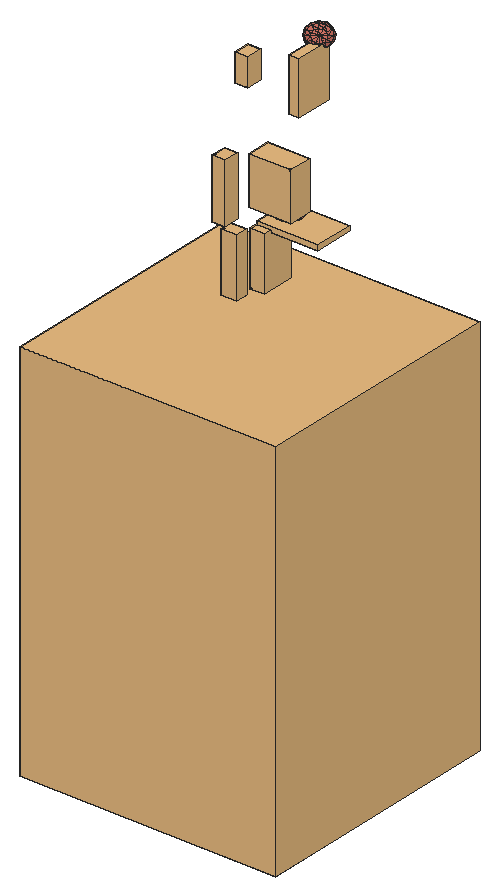
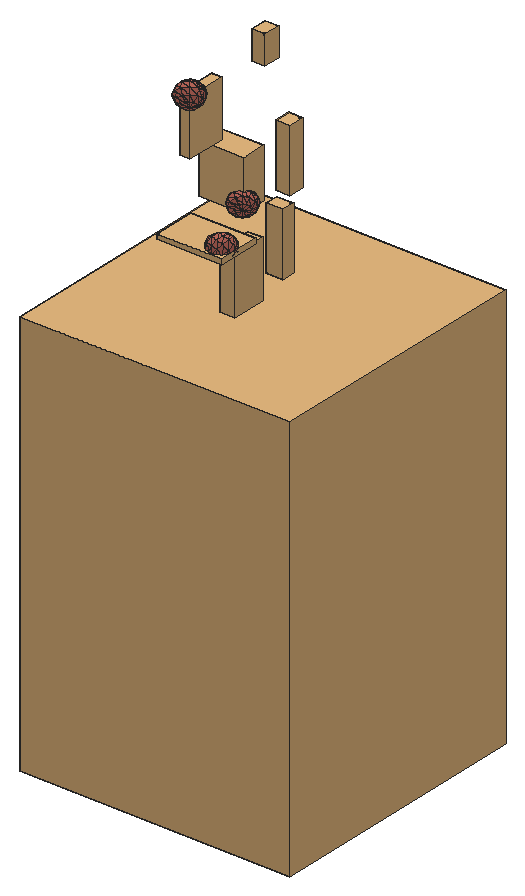
# SketchUp Ruby script. Lengths in inches.
U = 1.inch
M = Sketchup.active_model
def pt(a) = Geom::Point3d.new(a.map { |v| v * U })
def face(e, loops, mat)
  f = e.add_face(loops[0].map { |a| pt(a) })
  loops[1..].each { |l| e.add_face(l.map { |a| pt(a) }).erase! }
  f.material = f.back_material = mat if mat
  f
end
# faces: each face lists its corners as indices into pts; further lists are holes
def faces(e, pts, list, mat = nil) = list.each { |f| face(e, (f[0].is_a?(Array) ? f : [f]).map { |l| l.map { |i| pts[i] } }, mat) }
# xy, xz, yz: faces in a plane at the given z, y or x. An outline is a flat list of corners, or four numbers for a rectangle; further outlines are holes
def ring(l) = l.size == 4 ? [[l[0], l[1]], [l[2], l[1]], [l[2], l[3]], [l[0], l[3]]] : l.each_slice(2).to_a
def flat(e, list, mat, &to3) = list.each { |f| face(e, (f[0].is_a?(Array) ? f : [f]).map { |l| ring(l).map { |u, v| to3.(u, v) } }, mat) }
def xy(e, z, list, mat = nil) = flat(e, list, mat) { |x, y| [x, y, z] }
def xz(e, y, list, mat = nil) = flat(e, list, mat) { |x, z| [x, y, z] }
def yz(e, x, list, mat = nil) = flat(e, list, mat) { |y, z| [x, y, z] }
def lines(e, pts, list) = list.each { |a, b| e.add_line(pt(pts[a]), pt(pts[b])) }
# prism: a flat outline (further loops are holes) pulled along v
def prism(e, loops, v, mat = nil)
  f = face(e, loops, mat); d = Geom::Vector3d.new(v.map { |x| x * U })
  f.pushpull(f.normal.samedirection?(d) ? d.length : -d.length)
end
def box(e, o, s, mat = nil) = prism(e, [[o, [o[0] + s[0], o[1], o[2]], [o[0] + s[0], o[1] + s[1], o[2]], [o[0], o[1] + s[1], o[2]]]], [0, 0, s[2]], mat)
def at(x, y, z, deg = 0) = Geom::Transformation.translation(pt([x, y, z])) * Geom::Transformation.rotation(ORIGIN, Z_AXIS, deg.degrees)
def axes(o, x, y, z) = Geom::Transformation.new([*x, 0, *y, 0, *z, 0, *pt(o).to_a, 1])
def part(name) = M.definitions.add(name)
# library, detail: a bought-in or finely detailed component or shape, given as its bounding box
def library(name, o, s) = part(name).tap { |d| box(d.entities, o, s) }
def detail(e, o, s) = box(e.add_group.entities, o, s)
def put(e, d, t, mat = nil) = e.add_instance(d, t).tap { |i| i.material = mat if mat }
def group(e, t, mat = nil) = e.add_group.tap { |g| g.transformation = t; g.material = mat if mat }.entities
root = M.entities
M.materials.add("green").color = [174, 139, 102]
M.materials.add("st tile").color = [196, 179, 155]
M.materials.add("vio").color = [206, 114, 100]
c1 = library("3DGeom~165_Defintion",[-129.92,-500,-108.02],[259.84,1000,216.04])
c2 = part("3DGeom~166_Defintion")
p = [[102.48,500,-82.55],[119.68,491.3,-106.9],[111.55,493.01,-108.02],[102.48,500,-82.55],[111.55,493.01,-108.02],[104.2,495.34,-104.9],
  [102.48,500,-82.55],[126.4,490.68,-101.84],[119.68,491.3,-106.9],[102.48,500,-82.55],[104.2,495.34,-104.9],[99.59,497.67,-98.37],
  [102.48,500,-82.55],[129.92,491.3,-94.2],[126.4,490.68,-101.84],[102.48,500,-82.55],[99.59,497.67,-98.37],[98.96,499.375,-90.19],
  [102.48,500,-82.55],[129.29,493.01,-86.02],[129.92,491.3,-94.2],[102.48,500,-82.55],[124.6875,495.34,-79.5],[129.29,493.01,-86.02],
  [102.48,500,-82.55],[117.33,497.67,-76.375],[124.6875,495.34,-79.5],[102.48,500,-82.55],[109.21,499.375,-77.49],[117.33,497.67,-76.375],
  [-108.37,-495.57,69.37],[-118.11,-500,95.38],[-120.78,-498.52,79.375],[-93.3,-494.09,75.36],[-118.11,-500,95.38],[-108.37,-495.57,69.37],
  [-108.37,-495.57,69.37],[-120.78,-498.52,79.375],[-115.95,-497.04,72.67],[-93.3,-494.09,75.36],[-108.37,-495.57,69.37],[-100.08,-494.49,70.35],
  [-90.63,-495.57,91.37],[-118.11,-500,95.38],[-93.3,-494.09,75.36],[-90.63,-495.57,91.37],[-93.3,-494.09,75.36],[-89.84,-494.49,83.05],
  [-118.11,-500,95.38],[-121.57,-499.6,87.6875],[-120.78,-498.52,79.375],[-103.04,-498.52,101.375],[-118.11,-500,95.38],[-90.63,-495.57,91.37],
  [-103.04,-498.52,101.375],[-90.63,-495.57,91.37],[-95.46,-497.04,98.07],[-118.11,-500,95.38],[-103.04,-498.52,101.375],[-111.33,-499.6,100.39]]
faces(c2.entities,p,[[0,1,2],[3,4,5],[6,7,8],[9,10,11],[12,13,14],[15,16,17],[18,19,20],[21,22,23],
  [24,25,26],[27,28,29],[30,31,32],[33,34,35],[36,37,38],[39,40,41],[42,43,44],[45,46,47],
  [48,49,50],[51,52,53],[54,55,56],[57,58,59]],"green")
c3 = library("3DGeom~177_Defintion",[-102.18,-500,-134.58],[204.36,1000,269.16])
c4 = part("3DGeom~178_Defintion")
p = [[77.2,500,-106.58],[95.25,490.68,-131.46],[87.43,491.3,-134.58],[77.2,500,-106.58],[87.43,491.3,-134.58],[79.3,493.01,-133.53],
  [77.2,500,-106.58],[79.3,493.01,-133.53],[73.02,495.34,-128.6],[77.2,500,-106.58],[100.64,491.3,-125],[95.25,490.68,-131.46],
  [77.2,500,-106.58],[73.02,495.34,-128.6],[70.28,497.67,-121.1],[77.2,500,-106.58],[102.18,493.01,-116.9375],[100.64,491.3,-125],
  [77.2,500,-106.58],[70.28,497.67,-121.1],[71.81,499.375,-113.04],[77.2,500,-106.58],[99.43,495.34,-109.4375],[102.18,493.01,-116.9375],
  [77.2,500,-106.58],[93.15,497.67,-104.5],[99.43,495.34,-109.4375],[77.2,500,-106.58],[85.02,499.375,-103.46],[93.15,497.67,-104.5],
  [-70.48,-494.09,97.03],[-86.6,-495.57,95.18],[-78.34,-494.49,93.96],[-86.6,-495.57,95.18],[-89.2,-500,122.83],[-95.96,-498.52,108.09],
  [-70.48,-494.09,97.03],[-89.2,-500,122.83],[-86.6,-495.57,95.18],[-86.6,-495.57,95.18],[-95.96,-498.52,108.09],[-93.05,-497.04,100.35],
  [-63.72,-495.57,111.78],[-89.2,-500,122.83],[-70.48,-494.09,97.03],[-63.72,-495.57,111.78],[-70.48,-494.09,97.03],[-65.13,-494.49,103.55],
  [-89.2,-500,122.83],[-94.55,-499.6,116.32],[-95.96,-498.52,108.09],[-73.08,-498.52,124.68],[-89.2,-500,122.83],[-63.72,-495.57,111.78],
  [-73.08,-498.52,124.68],[-63.72,-495.57,111.78],[-66.63,-497.04,119.51],[-89.2,-500,122.83],[-73.08,-498.52,124.68],[-81.34,-499.6,125.9]]
faces(c4.entities,p,[[0,1,2],[3,4,5],[6,7,8],[9,10,11],[12,13,14],[15,16,17],[18,19,20],[21,22,23],
  [24,25,26],[27,28,29],[30,31,32],[33,34,35],[36,37,38],[39,40,41],[42,43,44],[45,46,47],
  [48,49,50],[51,52,53],[54,55,56],[57,58,59]],"green")
c5 = library("3DGeom~138_Defintion",[-301.73,-500,-131.06],[603.46,1000,262.12])
c6 = part("3DGeom~139_Defintion")
p = [[272.8,-500,-99.27],[285.64,-496.58,-110.875],[273.61,-494.75,-82.625],[285.64,-496.58,-110.875],[272.8,-500,-99.27],[278.1,-499.36,-106.75],
  [273.61,-494.75,-82.625],[285.64,-496.58,-110.875],[287.25,-486.08,-77.6],[285.64,-496.58,-110.875],[293.39,-492.38,-110.55],[299.28,-487.9,-105.84],
  [300.09,-482.66,-89.21],[285.64,-496.58,-110.875],[299.28,-487.9,-105.84],[287.25,-486.08,-77.6],[285.64,-496.58,-110.875],[300.09,-482.66,-89.21],
  [300.09,-482.66,-89.21],[299.28,-487.9,-105.84],[301.73,-484.35,-98.03],[272.8,-500,-99.27],[273.61,-494.75,-82.625],[271.16,-498.3125,-90.4375],
  [287.25,-486.08,-77.6],[300.09,-482.66,-89.21],[294.79,-483.3,-81.72],[273.61,-494.75,-82.625],[287.25,-486.08,-77.6],[279.5,-490.28,-77.93],
  [-291.23,494.98,97.6],[-301.04,485.9375,118.13],[-296.26,485.84,125.99],[-291.23,494.98,97.6],[-296.26,485.84,125.99],[-288.67,487.64,130.72],
  [-291.23,494.98,97.6],[-301.73,487.91,109.26],[-301.04,485.9375,118.13],[-291.23,494.98,97.6],[-288.67,487.64,130.72],[-280.29,490.86,131.0625],
  [-291.23,494.98,97.6],[-298.14,491.22,101.74],[-301.73,487.91,109.26],[-291.23,494.98,97.6],[-280.29,490.86,131.0625],[-273.38,494.625,126.92],
  [-291.23,494.98,97.6],[-273.38,494.625,126.92],[-269.79,497.9375,119.41],[-291.23,494.98,97.6],[-270.48,499.9,110.54],[-275.26,500,102.68],
  [-291.23,494.98,97.6],[-275.26,500,102.68],[-282.85,498.2,97.95],[-291.23,494.98,97.6],[-269.79,497.9375,119.41],[-270.48,499.9,110.54]]
faces(c6.entities,p,[[0,1,2],[3,4,5],[6,7,8],[9,10,11],[12,13,14],[15,16,17],[18,19,20],[21,22,23],
  [24,25,26],[27,28,29],[30,31,32],[33,34,35],[36,37,38],[39,40,41],[42,43,44],[45,46,47],
  [48,49,50],[51,52,53],[54,55,56],[57,58,59]],"green")
c7 = part("3DGeom~203_Defintion")
p = [[282.28,-215.46,-337.03],[49.88,-186.59,-454.85],[87.7,0,-500],[282.28,-215.46,-337.03],[325.95,0,-389.16],[-174.05,0,-476.86],
  [-195.89,107.73,-450.79],[49.88,186.59,-454.85],[325.95,0,-389.16],[-195.89,-107.73,-450.79],[-389.16,0,-325.95],[-389.16,0,-325.95],
  [162.97,-373.1875,-194.58],[-53.44,-323.1875,-331.49],[162.97,-373.1875,-194.58],[282.28,-215.46,-337.03],[325.95,0,-389.16],[282.28,215.46,-337.03],
  [-255.54,186.59,-379.57],[-255.54,186.59,-379.57],[-53.44,323.19,-331.49],[282.28,215.46,-337.03],[-53.44,323.19,-331.49],[-255.54,-186.59,-379.57],
  [-389.16,0,-325.95],[-255.54,186.59,-379.57],[-389.16,0,-325.95],[439.04,-186.59,-128.9],[282.28,-215.46,-337.03],[325.95,0,-389.16],
  [476.86,0,-174.05],[282.28,215.46,-337.03],[-194.58,-373.1875,-162.97],[-337.03,-215.46,-282.28],[-255.54,-186.59,-379.57],[-255.54,-186.59,-379.57],
  [-53.44,-323.1875,-331.49],[-255.54,-186.59,-379.57],[-337.03,-215.46,-282.28],[-389.16,0,-325.95],[-337.03,215.46,-282.28],[-255.54,186.59,-379.57],
  [-53.44,323.19,-331.49],[-255.54,186.59,-379.57],[-337.03,215.46,-282.28],[335.72,-323.19,-5.54],[162.97,-373.1875,-194.58],[439.04,186.59,-128.9],
  [162.97,373.1875,-194.58],[282.28,215.46,-337.03],[-53.44,323.19,-331.49],[162.97,373.1875,-194.58],[0,-430.92,0],[-53.44,-323.1875,-331.49],
  [-53.44,-323.1875,-331.49],[162.97,-373.1875,-194.58],[-337.03,215.46,-282.28],[-194.58,373.1875,-162.97],[162.97,373.1875,-194.58],[-418.51,-186.59,-184.99],
  [-478.17,-107.73,-113.77],[-500,0,-87.7],[-478.17,107.73,-113.77],[-418.51,186.59,-184.99],[-335.72,-323.19,5.54],[-194.58,-373.1875,-162.97],
  [-335.72,-323.19,5.54],[-194.58,373.1875,-162.97],[194.58,-373.1875,162.97],[162.97,-373.1875,-194.58],[162.97,-373.1875,-194.58],[335.72,-323.19,-5.54],
  [162.97,373.1875,-194.58],[335.72,323.19,-5.54],[335.72,323.19,-5.54],[0,430.92,0],[-439.04,-186.59,128.9],[-335.72,-323.19,5.54],
  [-335.72,323.19,5.54],[-194.58,373.1875,-162.97],[478.17,-107.73,113.77],[500,0,87.7],[-162.97,-373.1875,194.58],[-335.72,-323.19,5.54],
  [-335.72,323.19,5.54],[418.51,-186.59,184.99],[478.17,107.73,113.77],[-476.86,0,174.05],[-439.04,186.59,128.9],[337.03,-215.46,282.28],
  [194.58,-373.1875,162.97],[418.51,186.59,184.99],[194.58,373.1875,162.97],[335.72,323.19,-5.54],[194.58,373.1875,162.97],[53.44,-323.19,331.49],
  [-335.72,323.19,5.54],[-162.97,373.1875,194.58],[-162.97,373.1875,194.58],[-282.28,-215.46,337.03],[-335.72,-323.19,5.54],[-162.97,-373.1875,194.58],
  [-282.28,-215.46,337.03],[-335.72,-323.19,5.54],[-162.97,373.1875,194.58],[389.16,0,325.95],[-325.95,0,389.16],[-282.28,-215.46,337.03],
  [-325.95,0,389.16],[-282.28,215.46,337.03],[-162.97,373.1875,194.58],[-282.28,215.46,337.03],[255.54,-186.59,379.57],[255.54,-186.59,379.57],
  [337.03,-215.46,282.28],[194.58,373.1875,162.97],[337.03,215.46,282.28],[337.03,215.46,282.28],[53.44,323.19,331.49],[-162.97,373.1875,194.58],
  [53.44,323.19,331.49],[-282.28,215.46,337.03],[-325.95,0,389.16],[-49.88,-186.59,454.85],[-282.28,-215.46,337.03],[-162.97,-373.1875,194.58],
  [-162.97,-373.1875,194.58],[53.44,-323.19,331.49],[53.44,323.19,331.49],[-162.97,373.1875,194.58],[-282.28,215.46,337.03],[255.54,-186.59,379.57],
  [255.54,186.59,379.57],[337.03,215.46,282.28],[53.44,323.19,331.49],[255.54,186.59,379.57],[195.89,-107.73,450.79],[255.54,-186.59,379.57],
  [389.16,0,325.95],[174.05,0,476.86],[389.16,0,325.95],[195.89,107.73,450.79],[389.16,0,325.95],[255.54,186.59,379.57],
  [389.16,0,325.95],[53.44,-323.19,331.49],[53.44,-323.19,331.49],[255.54,-186.59,379.57],[-49.88,186.59,454.85],[-87.7,0,500],
  [-325.95,0,389.16]]
faces(c7.entities,p,[[0,1,2],[3,2,4],[1,5,2],[2,5,6],[2,6,7],[8,2,7],[1,9,5],[5,9,10],
  [6,5,11],[12,13,1],[14,1,15],[13,9,1],[16,7,17],[7,6,18],[7,19,20],[21,7,22],
  [13,23,9],[9,23,24],[25,6,26],[27,28,29],[27,29,30],[30,29,31],[32,33,34],[32,35,36],
  [37,38,39],[40,41,39],[42,43,44],[45,46,28],[45,28,27],[30,31,47],[47,31,48],[49,50,51],
  [52,32,53],[52,54,55],[42,56,57],[58,42,57],[38,59,39],[59,60,39],[60,61,39],[61,62,39],
  [62,63,39],[63,40,39],[64,38,65],[66,59,38],[67,40,63],[68,52,69],[68,70,71],[47,72,73],
  [74,58,75],[58,57,75],[76,59,77],[76,60,59],[78,63,62],[79,63,78],[80,27,30],[80,30,81],
  [81,30,47],[82,32,52],[82,83,32],[75,57,84],[85,45,27],[85,27,80],[81,47,86],[86,47,73],
  [87,60,76],[87,61,60],[88,62,61],[78,62,88],[88,61,87],[89,90,45],[89,45,85],[86,73,91],
  [91,73,92],[93,75,94],[95,82,52],[95,52,68],[75,96,97],[94,75,98],[99,100,101],[102,76,103],
  [104,78,88],[80,81,105],[81,86,105],[85,80,105],[86,91,105],[106,76,107],[108,87,76],[109,88,87],
  [110,88,111],[112,95,68],[113,68,114],[91,115,116],[117,94,118],[94,119,120],[121,87,122],[89,85,105],
  [91,116,105],[123,124,125],[123,126,127],[128,129,130],[131,89,105],[116,132,105],[133,134,135],[136,137,138],
  [139,136,140],[141,139,142],[143,141,144],[136,123,145],[136,146,147],[128,130,148],[143,128,148],[149,150,124],
  [149,124,123],[148,130,150],[143,148,141],[148,150,149],[139,123,136],[141,148,149],[141,149,139],[139,149,123]],"vio")
c8 = library("3DGeom~86_Defintion",[-294.02,-500,-230.29],[588.04,1000,460.58])
c9 = part("3DGeom~87_Defintion")
p = [[-277.25,494.74,-178.13],[-259.65,461.52,-230.29],[-276.72,461.46,-224.28],[-277.25,494.74,-178.13],[-242.66,466.72,-229.15],[-277.25,494.74,-178.13],
  [-230.3,475.68,-221.18],[-277.25,494.74,-178.13],[-276.72,461.46,-224.28],[-289.3,466.57,-212.75],[-277.25,494.74,-178.13],[-225.89,485.99,-208.51],
  [-230.3,475.68,-221.18],[-277.25,494.74,-178.13],[-289.3,466.57,-212.75],[-294.02,475.47,-198.77],[-277.25,494.74,-178.13],[-230.61,494.89,-194.54],
  [-225.89,485.99,-208.51],[-277.25,494.74,-178.13],[-294.02,475.47,-198.77],[-289.61,485.79,-186.1],[-277.25,494.74,-178.13],[-243.1875,500,-183],
  [-230.61,494.89,-194.54],[-277.25,494.74,-178.13],[-260.26,499.95,-177],[-243.1875,500,-183],[274.19,-487.18,163.98],[243.1875,-498.77,172.64],
  [258.02,-494.08,163.86],[274.19,-487.18,163.98],[251.86,-484.5,230.17],[243.1875,-498.77,172.64],[294.02,-474.24,188.41],[251.86,-484.5,230.17],
  [274.19,-487.18,163.98],[294.02,-474.24,188.41],[274.19,-487.18,163.98],[287.36,-479.92,172.97],[243.1875,-498.77,172.64],[232.02,-497.43,205.74],
  [233.67,-500,187.97],[243.1875,-498.77,172.64],[251.86,-484.5,230.17],[232.02,-497.43,205.74],[282.85,-472.9,221.51],[251.86,-484.5,230.17],
  [294.02,-474.24,188.41],[282.85,-472.9,221.51],[294.02,-474.24,188.41],[292.37,-471.67,206.18],[251.86,-484.5,230.17],[238.68,-491.76,221.18],
  [232.02,-497.43,205.74],[251.86,-484.5,230.17],[282.85,-472.9,221.51],[268.02,-477.6,230.29]]
faces(c9.entities,p,[[0,1,2],[3,4,1],[5,6,4],[7,8,9],[10,11,12],[13,14,15],[16,17,18],[19,20,21],
  [22,23,24],[25,26,27],[28,29,30],[31,32,33],[34,35,36],[37,38,39],[40,41,42],[43,44,45],
  [46,47,48],[49,50,51],[52,53,54],[55,56,57]],"green")
c10 = part("3DGeom~231_Defintion")
p = [[55.77,-247.26,-406.4],[-282.99,-160.1875,-370.7],[-76.91,-70.8125,-490.14],[264.6875,-115.27,-405.72],[-380.05,9.05,-329.48],[149.78,37.54,-478.25],
  [-188.98,124.61,-442.55],[402.68,47.61,-296.34],[52.72,206.77,-437.03],[336.34,135.83,-338.21],[402.68,47.61,-296.34],[336.34,135.83,-338.21],
  [-433.25,149.375,-185.58],[-433.25,149.375,-185.58],[-250.42,286.64,-276.38],[-250.42,286.64,-276.38],[336.34,135.83,-338.21],[280.3,233.54,-314.41],
  [-250.42,286.64,-276.38],[-0.48,347.1,-293.125],[280.3,233.54,-314.41],[-0.48,347.1,-293.125],[173.51,-357.45,-213.76],[-168.09,-312.99,-298.18],
  [55.77,-247.26,-406.4],[366.65,-210.7,-238.9],[173.51,-357.45,-213.76],[-168.09,-312.99,-298.18],[366.65,-210.7,-238.9],[461.55,-7.49,-200.02],
  [366.65,-210.7,-238.9],[264.6875,-115.27,-405.72],[264.6875,-115.27,-405.72],[402.68,47.61,-296.34],[-168.09,-312.99,-298.18],[-413.24,-206.64,-151.93],
  [-282.99,-160.1875,-370.7],[-282.99,-160.1875,-370.7],[-469.28,-108.93,-128.14],[-282.99,-160.1875,-370.7],[-380.05,9.05,-329.48],[336.34,135.83,-338.21],
  [432.77,197.72,-107.55],[280.3,233.54,-314.41],[-380.05,9.05,-329.48],[-500,-27.91,-45.05],[-380.05,9.05,-329.48],[-433.25,149.375,-185.58],
  [249.58,314.55,-231.33],[280.3,233.54,-314.41],[-0.48,347.1,-293.125],[249.58,314.55,-231.33],[-66.125,-408.42,-131.35],[-346.9,-294.86,-110.06],
  [-168.09,-312.99,-298.18],[173.51,-357.45,-213.76],[-168.09,-312.99,-298.18],[-168.09,-312.99,-298.18],[-346.9,-294.86,-110.06],[-0.48,347.1,-293.125],
  [-250.42,286.64,-276.38],[-244.75,371.86,-36.15],[249.58,314.55,-231.33],[4.42,420.91,-85.08],[-250.42,286.64,-276.38],[-428.35,223.18,22.47],
  [-250.42,286.64,-276.38],[-244.75,371.86,-36.15],[428.35,-223.18,-22.47],[173.51,-357.45,-213.76],[497.17,-14.7,-75.0625],[252.41,357.17,-111.21],
  [249.58,314.55,-231.33],[252.41,357.17,-111.21],[244.75,-371.86,36.15],[173.51,-357.45,-213.76],[244.75,-371.86,36.15],[173.51,-357.45,-213.76],
  [-497.17,14.7,75.0625],[-432.77,-197.72,107.55],[-4.42,-420.91,85.08],[-288.04,-349.96,-13.74],[244.75,-371.86,36.15],[-346.9,-294.86,-110.06],
  [288.04,349.96,13.74],[252.41,357.17,-111.21],[66.12,408.42,131.35],[288.04,349.96,13.74],[252.41,357.17,-111.21],[-288.04,-349.96,-13.74],
  [500,27.91,45.05],[469.28,108.93,128.14],[413.24,206.64,151.93],[346.9,294.86,110.06],[-173.51,357.45,213.76],[-244.75,371.86,-36.15],
  [-366.65,210.7,238.9],[-244.75,371.86,-36.15],[-366.65,210.7,238.9],[-173.51,357.45,213.76],[433.25,-149.375,185.58],[-252.41,-357.17,111.22],
  [-288.04,-349.96,-13.74],[-252.41,-357.17,111.22],[288.04,349.96,13.74],[168.09,312.99,298.18],[346.9,294.86,110.06],[288.04,349.96,13.74],
  [168.09,312.99,298.18],[-461.55,7.49,200.02],[-366.65,210.7,238.9],[250.42,-286.64,276.38],[244.75,-371.86,36.15],[250.42,-286.64,276.38],
  [0.48,-347.1,293.125],[250.42,-286.64,276.38],[-252.41,-357.17,111.22],[-249.58,-314.55,231.33],[-249.58,-314.55,231.33],[-280.3,-233.54,314.41],
  [-280.3,-233.54,314.41],[-336.34,-135.83,338.21],[-402.68,-47.6,296.34],[-336.34,-135.83,338.21],[-402.68,-47.6,296.34],[168.09,312.99,298.18],
  [282.99,160.1875,370.7],[-249.58,-314.55,231.33],[380.05,-9.05,329.48],[-55.77,247.26,406.4],[-55.77,247.26,406.4],[168.09,312.99,298.18],
  [380.05,-9.05,329.48],[250.42,-286.64,276.38],[433.25,-149.375,185.58],[-366.65,210.7,238.9],[-402.68,-47.6,296.34],[-173.51,357.45,213.76],
  [-366.65,210.7,238.9],[-264.6875,115.27,405.72],[-173.51,357.45,213.76],[-55.77,247.26,406.4],[-52.72,-206.77,437.03],[-249.58,-314.55,231.33],
  [0.48,-347.1,293.125],[-280.3,-233.54,314.41],[-249.58,-314.55,231.33],[-366.65,210.7,238.9],[-402.68,-47.6,296.34],[-264.6875,115.27,405.72],
  [188.98,-124.61,442.55],[0.48,-347.1,293.125],[250.42,-286.64,276.38],[380.05,-9.05,329.48],[250.42,-286.64,276.38],[0.48,-347.1,293.125],
  [-402.68,-47.6,296.34],[-336.34,-135.83,338.21],[168.09,312.99,298.18],[76.91,70.8125,490.14],[168.09,312.99,298.18],[282.99,160.1875,370.7],
  [-149.78,-37.54,478.25],[282.99,160.1875,370.7],[380.05,-9.05,329.48],[282.99,160.1875,370.7]]
faces(c10.entities,p,[[0,1,2],[3,0,2],[2,1,4],[3,2,5],[2,4,6],[5,2,6],[7,3,5],[5,6,8],
  [9,5,8],[10,5,11],[6,4,12],[6,13,14],[8,6,15],[16,8,17],[8,18,19],[20,8,21],
  [22,23,24],[25,26,0],[0,27,1],[28,0,3],[29,30,31],[29,32,33],[34,35,36],[37,35,38],
  [39,38,40],[33,41,42],[41,43,42],[44,38,45],[46,45,47],[43,48,42],[49,50,51],[52,53,54],
  [55,52,56],[57,58,35],[29,33,42],[59,60,61],[62,59,63],[59,61,63],[64,47,65],[66,65,67],
  [68,69,30],[70,68,30],[70,30,29],[48,71,42],[72,63,73],[74,52,75],[68,76,77],[70,29,42],
  [47,45,78],[47,78,65],[35,58,79],[38,35,79],[80,81,52],[82,80,52],[52,81,83],[45,38,79],
  [71,84,42],[85,86,87],[88,63,86],[58,89,79],[90,70,42],[91,90,42],[92,91,42],[84,93,42],
  [93,92,42],[63,61,94],[63,94,86],[90,68,70],[78,45,79],[95,65,96],[97,98,99],[100,76,68],
  [90,100,68],[80,101,81],[102,103,79],[104,105,106],[107,86,108],[65,78,109],[65,109,110],[111,80,112],
  [100,113,76],[91,100,90],[109,78,79],[114,101,80],[115,114,80],[116,117,79],[118,119,79],[120,121,79],
  [122,109,79],[123,124,79],[93,125,126],[93,126,92],[114,127,101],[91,128,100],[92,128,91],[86,94,129],
  [86,130,131],[92,126,128],[132,133,134],[135,109,136],[137,138,139],[140,139,141],[142,143,144],[142,145,146],
  [147,148,149],[150,151,152],[153,150,154],[150,142,155],[139,156,157],[158,141,159],[160,159,161],[162,157,145],
  [162,145,142],[163,150,164],[139,157,162],[165,159,150],[141,139,162],[141,162,159],[159,162,142],[159,142,150]],"vio")
c11 = part("3DGeom~201_Defintion")
p = [[110.02,-100.74,-478.98],[-201.3,-79.76,-454.16],[-6.43,63.34,-500],[324.63,0,-387.59],[-294.01,-10.41,-411.12],[-167.01,183.46,-425.45],
  [324.63,0,-387.59],[190.15,189.47,-411.86],[190.15,189.47,-411.86],[151.15,-264.83,-368.01],[-134.06,-174.49,-442.02],[372.12,-189.47,-259.46],
  [372.12,-189.47,-259.46],[324.63,0,-387.59],[-342.22,-201.49,-286.63],[-342.22,-201.49,-286.63],[-110.3125,-269.23,-377.96],[-342.22,-201.49,-286.63],
  [-387.35,14.98,-324.43],[-387.35,14.98,-324.43],[-328.69,227.43,-275.3],[4.73,328.17,-325.78],[-328.69,227.43,-275.3],[190.15,189.47,-411.86],
  [4.73,328.17,-325.78],[452.25,100.74,-192.35],[324.63,0,-387.59],[190.15,189.47,-411.86],[190.15,189.47,-411.86],[335.79,264.83,-213.37],
  [335.79,264.83,-213.37],[190.15,189.47,-411.86],[4.73,328.17,-325.78],[-387.35,14.98,-324.43],[-294.01,-10.41,-411.12],[-342.22,-201.49,-286.63],
  [493.375,-63.34,-81.39],[372.12,-189.47,-259.46],[105.93,-384.95,-196.84],[-136.42,-338.58,-279.13],[-110.3125,-269.23,-377.96],[-110.3125,-269.23,-377.96],
  [151.15,-264.83,-368.01],[-136.42,-338.58,-279.13],[-342.22,-201.49,-286.63],[319.9,-328.17,-61.81],[151.15,-264.83,-368.01],[319.9,-328.17,-61.81],
  [151.15,-264.83,-368.01],[372.12,-189.47,-259.46],[4.73,328.17,-325.78],[-328.69,227.43,-275.3],[-181.96,378.94,-152.4],[175.21,384.95,-138.82],
  [-181.96,378.94,-152.4],[-456.32,-10.41,-217.32],[-328.69,227.43,-275.3],[-205.39,-363.96,-172.03],[-342.22,-201.49,-286.63],[-205.39,-363.96,-172.03],
  [-298.74,-338.58,-85.34],[-298.74,-338.58,-85.34],[-391.45,-269.23,-42.3],[-391.45,-269.23,-42.3],[-458.6875,-174.49,-54.43],[-482.43,-79.76,-118.5],
  [-13.53,-428.92,-11.33],[-448.15,183.46,-89.79],[-181.96,378.94,-152.4],[448.15,-183.46,89.79],[319.9,-328.17,-61.81],[458.6875,174.49,54.43],
  [335.79,264.83,-213.37],[335.79,264.83,-213.37],[391.45,269.23,42.3],[391.45,269.23,42.3],[181.96,-378.94,152.4],[181.96,-378.94,152.4],
  [319.9,-328.17,-61.81],[482.43,79.76,118.5],[-175.21,-384.95,138.82],[-298.74,-338.58,-85.34],[-181.96,378.94,-152.4],[-319.9,328.17,61.81],
  [13.53,428.92,11.33],[-319.9,328.17,61.81],[391.45,269.23,42.3],[298.74,338.58,85.34],[298.74,338.58,85.34],[-493.375,63.34,81.38],
  [-319.9,328.17,61.81],[-335.79,-264.83,213.37],[-391.45,-269.23,-42.3],[456.32,10.41,217.32],[328.69,-227.43,275.3],[181.96,-378.94,152.4],
  [328.69,-227.43,275.3],[-452.25,-100.74,192.35],[-391.45,-269.23,-42.3],[-391.45,-269.23,-42.3],[-335.79,-264.83,213.37],[-4.73,-328.17,325.78],
  [-4.73,-328.17,325.78],[181.96,-378.94,152.4],[-105.93,384.95,196.84],[298.74,338.58,85.34],[205.39,363.96,172.03],[342.22,201.49,286.63],
  [298.74,338.58,85.34],[-319.9,328.17,61.81],[-372.12,189.47,259.46],[-372.12,189.47,259.46],[-372.12,189.47,259.46],[205.39,363.96,172.03],
  [387.35,-14.98,324.43],[328.69,-227.43,275.3],[-190.15,-189.47,411.86],[-190.15,-189.47,411.86],[-4.73,-328.17,325.78],[167.01,-183.46,425.45],
  [-4.73,-328.17,325.78],[181.96,-378.94,152.4],[328.69,-227.43,275.3],[136.42,338.58,279.13],[342.22,201.49,286.63],[136.42,338.58,279.13],
  [-324.63,0,387.59],[-335.79,-264.83,213.37],[-372.12,189.47,259.46],[-324.63,0,387.59],[-372.12,189.47,259.46],[-151.15,264.83,368.01],
  [136.42,338.58,279.13],[-151.15,264.83,368.01],[-324.63,0,387.59],[-335.79,-264.83,213.37],[-190.15,-189.47,411.86],[-151.15,264.83,368.01],
  [-372.12,189.47,259.46],[-324.63,0,387.59],[294.01,10.41,411.12],[294.01,10.41,411.12],[387.35,-14.98,324.43],[136.42,338.58,279.13],
  [110.3125,269.23,377.96],[342.22,201.49,286.63],[136.42,338.58,279.13],[-151.15,264.83,368.01],[110.3125,269.23,377.96],[294.01,10.41,411.12],
  [201.3,79.76,454.16],[294.01,10.41,411.12],[342.22,201.49,286.63],[134.06,174.49,442.02],[342.22,201.49,286.63],[342.22,201.49,286.63],
  [6.43,-63.34,500],[-190.15,-189.47,411.86],[-110.03,100.74,478.98],[294.01,10.41,411.12]]
faces(c11.entities,p,[[0,1,2],[3,0,2],[2,1,4],[2,4,5],[6,2,7],[8,2,5],[9,10,0],[11,9,0],
  [12,0,13],[0,10,1],[4,1,14],[1,10,15],[10,16,17],[9,16,10],[5,4,18],[5,19,20],
  [21,5,22],[23,5,24],[25,26,27],[25,28,29],[30,31,32],[33,34,35],[36,37,26],[36,26,25],
  [38,39,40],[38,41,42],[16,43,44],[45,38,46],[47,48,49],[50,51,52],[30,32,53],[53,32,54],
  [55,33,35],[56,33,55],[39,57,58],[59,60,35],[61,62,35],[63,64,35],[64,65,35],[65,55,35],
  [66,57,39],[66,39,38],[56,55,67],[68,56,67],[69,70,37],[69,37,36],[67,55,65],[71,25,72],
  [71,73,74],[75,30,53],[76,66,38],[77,38,78],[79,36,25],[79,25,71],[80,57,66],[80,81,57],
  [82,67,83],[84,54,85],[53,54,84],[86,53,87],[88,53,84],[89,65,64],[67,65,89],[90,67,89],
  [91,81,80],[91,92,81],[93,69,36],[93,36,79],[94,95,70],[96,70,69],[97,64,98],[89,64,97],
  [97,99,100],[101,80,66],[102,66,103],[84,85,104],[105,84,106],[106,84,104],[71,74,107],[74,108,107],
  [79,71,107],[109,89,110],[104,85,111],[112,89,97],[108,113,107],[114,115,69],[114,69,93],[93,79,107],
  [116,91,80],[117,80,118],[119,120,121],[119,121,122],[106,123,124],[106,104,125],[126,97,127],[128,97,129],
  [104,130,131],[132,104,133],[134,135,136],[114,93,107],[137,138,139],[140,119,122],[141,122,142],[143,144,145],
  [146,147,148],[149,114,107],[150,151,152],[153,150,154],[144,153,155],[156,157,120],[156,120,119],[137,139,158],
  [144,137,158],[144,158,153],[158,139,157],[150,119,159],[158,157,156],[150,156,119],[153,158,156],[153,156,150]],"vio")
c12 = library("3DGeom~51_Defintion",[-354.35,-500,-93.25],[708.7,1000,186.5])
c13 = part("3DGeom~52_Defintion")
p = [[-330.32,495.99,-90.07],[-337.71,491.72,-93.25],[-345.49,487.36,-91.53],[-330.32,495.99,-90.07],[-345.49,487.36,-91.53],[-351.58,484.07,-85.375],
  [-330.32,495.99,-90.07],[-351.58,484.07,-85.375],[-354.35,482.74,-76.44],[-330.32,495.99,-90.07],[-354.35,482.74,-76.44],[-353.05,483.72,-67.125],
  [-330.32,495.99,-90.07],[-353.05,483.72,-67.125],[-348.04,486.75,-59.91],[-330.32,495.99,-90.07],[-348.04,486.75,-59.91],[-340.65,491.02,-56.74],
  [-330.32,495.99,-90.07],[-340.65,491.02,-56.74],[-332.87,495.38,-58.46],[-330.32,495.99,-90.07],[-332.87,495.38,-58.46],[-326.78,498.67,-64.61],
  [-330.32,495.99,-90.07],[-326.78,498.67,-64.61],[-324.02,500,-73.54],[-330.32,495.99,-90.07],[-324.02,500,-73.54],[-325.3125,499.02,-82.86],
  [349.875,-495.14,64.65],[332.69,-500,61.93],[341.95,-498.4,61.14],[332.69,-500,61.93],[349.875,-495.14,64.65],[319.79,-497.07,74.47],
  [332.69,-500,61.93],[319.79,-497.07,74.47],[324.58,-499.51,66.81],[319.79,-497.07,74.47],[349.875,-495.14,64.65],[324.08,-489.29,89.73],
  [324.08,-489.29,89.73],[349.875,-495.14,64.65],[341.27,-484.43,92.46],[341.27,-484.43,92.46],[349.875,-495.14,64.65],[354.16,-487.36,79.92],
  [349.875,-495.14,64.65],[354.35,-491.1,71.52],[354.16,-487.36,79.92],[319.79,-497.07,74.47],[324.08,-489.29,89.73],[319.61,-493.33,82.86],
  [341.27,-484.43,92.46],[354.16,-487.36,79.92],[349.38,-484.91,87.58],[324.08,-489.29,89.73],[341.27,-484.43,92.46],[332.01,-486.03,93.25]]
faces(c13.entities,p,[[0,1,2],[3,4,5],[6,7,8],[9,10,11],[12,13,14],[15,16,17],[18,19,20],[21,22,23],
  [24,25,26],[27,28,29],[30,31,32],[33,34,35],[36,37,38],[39,40,41],[42,43,44],[45,46,47],
  [48,49,50],[51,52,53],[54,55,56],[57,58,59]],"green")
c14 = library("3DGeom~187_Defintion",[-331.51,-500,-331.51],[663.02,1000,663.02])
c15 = library("3DGeom~49_Defintion",[-249.27,-500,-442.2],[498.54,1000,884.4])
c16 = part("3DGeom~50_Defintion")
p = [[-222.48,-492.22,-439.3125],[-238.52,-481.53,-439.75],[-230.08,-486.5,-442.2],[-238.52,-481.53,-439.75],[-222.48,-492.22,-439.3125],[-249.27,-478.62,-422.75],
  [-238.52,-481.53,-439.75],[-249.27,-478.62,-422.75],[-245.54,-478.65,-432.64],[-227.92,-497.09,-404.87],[-222.48,-492.22,-439.3125],[-217.17,-500,-421.87],
  [-222.48,-492.22,-439.3125],[-217.75,-497.16,-431.875],[-217.17,-500,-421.87],[-243.96,-486.4,-405.31],[-222.48,-492.22,-439.3125],[-227.92,-497.09,-404.87],
  [-249.27,-478.62,-422.75],[-222.48,-492.22,-439.3125],[-243.96,-486.4,-405.31],[-249.27,-478.62,-422.75],[-243.96,-486.4,-405.31],[-248.6875,-481.46,-412.75],
  [-227.92,-497.09,-404.87],[-217.17,-500,-421.87],[-220.89,-499.97,-411.99],[-243.96,-486.4,-405.31],[-227.92,-497.09,-404.87],[-236.36,-492.12,-402.43],
  [245.19,493.0625,414.62],[236.94,497.78,411.0625],[226.73,500,411.68],[245.19,493.0625,414.62],[226.73,500,411.68],[217.29,499.13,416.31],
  [245.19,493.0625,414.62],[222.29,479.16,442.2],[232.5,476.9375,441.58],[245.19,493.0625,414.62],[241.9375,477.81,436.95],[245.19,493.0625,414.62],
  [241.9375,477.81,436.95],[248.08,481.53,429.5625],[245.19,493.0625,414.62],[214.04,483.875,438.65],[245.19,493.0625,414.62],[248.08,481.53,429.5625],
  [249.27,487.12,421.39],[245.19,493.0625,414.62],[209.96,489.82,431.875],[245.19,493.0625,414.62],[211.15,495.41,423.7],[209.96,489.82,431.875],
  [245.19,493.0625,414.62],[217.29,499.13,416.31],[211.15,495.41,423.7]]
faces(c16.entities,p,[[0,1,2],[3,4,5],[6,7,8],[9,10,11],[12,13,14],[15,16,17],[18,19,20],[21,22,23],
  [24,25,26],[27,28,29],[30,31,32],[33,34,35],[36,37,38],[39,38,40],[41,42,43],[44,45,37],
  [46,47,48],[49,50,45],[51,52,53],[54,55,56]],"green")
c17 = library("3DGeom~63_Defintion",[-323.2,-41,-500],[646.4,82,1000])
c18 = part("3DGeom~64_Defintion")
p = [[311.67,-40.04,-491.9],[306.7,-29.34,-500],[319.92,-38.4,-478.58],[306.7,-29.34,-500],[311.67,-40.04,-491.9],[308.29,-35.77,-497.38],
  [319.92,-38.4,-478.58],[306.7,-29.34,-500],[323.2,-26.06,-473.36],[306.7,-29.34,-500],[307.3125,-22.47,-499.05],[309.97,-17,-494.78],
  [318.22,-15.36,-481.47],[306.7,-29.34,-500],[309.97,-17,-494.78],[323.2,-26.06,-473.36],[306.7,-29.34,-500],[318.22,-15.36,-481.47],
  [318.22,-15.36,-481.47],[309.97,-17,-494.78],[313.97,-14.4,-488.35],[311.67,-40.04,-491.9],[319.92,-38.4,-478.58],[315.93,-41,-485.02],
  [323.2,-26.06,-473.36],[318.22,-15.36,-481.47],[321.6,-19.63,-475.98],[319.92,-38.4,-478.58],[323.2,-26.06,-473.36],[322.58,-32.93,-474.31],
  [-323.2,26.33,486.21],[-308.11,14.4,494.77],[-301.1875,16.87,498],[-323.2,26.33,486.21],[-315.3,15.5,491.1],[-308.11,14.4,494.77],
  [-323.2,26.33,486.21],[-320.82,19.86,487.96],[-315.3,15.5,491.1],[-323.2,26.33,486.21],[-301.1875,16.87,498],[-296.38,22.24,499.91],
  [-323.2,26.33,486.21],[-296.38,22.24,499.91],[-294.98,29.07,500],[-323.2,26.33,486.21],[-310.07,41,491.4375],[-316.99,38.53,488.21],
  [-323.2,26.33,486.21],[-316.99,38.53,488.21],[-321.8,33.16,486.3],[-323.2,26.33,486.21],[-297.36,35.54,498.24],[-302.88,39.9,495.11],
  [-323.2,26.33,486.21],[-302.88,39.9,495.11],[-310.07,41,491.4375],[-323.2,26.33,486.21],[-294.98,29.07,500],[-297.36,35.54,498.24]]
faces(c18.entities,p,[[0,1,2],[3,4,5],[6,7,8],[9,10,11],[12,13,14],[15,16,17],[18,19,20],[21,22,23],
  [24,25,26],[27,28,29],[30,31,32],[33,34,35],[36,37,38],[39,40,41],[42,43,44],[45,46,47],
  [48,49,50],[51,52,53],[54,55,56],[57,58,59]],"green")
g1 = group(root,at(15.3125,134.49,26.21))
put(g1,c1,axes([-0.88,-0.16,7.92],[0,0.00091,0],[0,0,-0.00091],[-0.00091,0,0]),"green")
put(g1,c2,axes([-0.88,-0.16,7.92],[0,0.00091,0],[0,0,-0.00091],[-0.00091,0,0]),"green")
g2 = group(root,at(15.3125,134.49,26.21))
put(g2,c3,axes([-0.83,-0.05,6.86],[0,0.00091,0],[0,0,-0.00091],[-0.00091,0,0]),"green")
put(g2,c4,axes([-0.83,-0.05,6.86],[0,0.00091,0],[0,0,-0.00091],[-0.00091,0,0]),"green")
g3 = group(root,at(15.3125,134.49,26.21))
put(g3,c5,axes([-0.82,0.64,6.68],[0,0.00083,0],[0,0,-0.00083],[-0.00083,0,0]),"green")
put(g3,c6,axes([-0.82,0.64,6.68],[0,0.00083,0],[0,0,-0.00083],[-0.00083,0,0]),"green")
g4 = group(root,at(15.3125,134.49,26.21))
put(g4,c7,axes([-0.82,0.61,7.6],[0,0.00038,0],[0,0,-0.00038],[-0.00038,0,0]),"vio")
g5 = group(root,at(15.3125,134.49,26.21))
put(g5,c8,axes([-0.79,0.17,9.47],[0,0.00042,0],[0,0,-0.00042],[-0.00042,0,0]),"green")
put(g5,c9,axes([-0.79,0.17,9.47],[0,0.00042,0],[0,0,-0.00042],[-0.00042,0,0]),"green")
g6 = group(root,at(15.3125,134.49,26.21))
put(g6,c10,axes([-0.74,0.9,7.125],[0,0.00039,0],[0,0,-0.00039],[-0.00039,0,0]),"vio")
g7 = group(root,at(15.3125,134.49,26.21))
put(g7,c11,axes([-0.73,1.46,9.35],[0,0.00039,0],[0,0,-0.00039],[-0.00039,0,0]),"vio")
g8 = group(root,at(15.3125,134.49,26.21))
put(g8,c12,axes([-0.66,1.17,8.92],[0,0.00081,0],[0,0,-0.00081],[-0.00081,0,0]),"green")
put(g8,c13,axes([-0.66,1.17,8.92],[0,0.00081,0],[0,0,-0.00081],[-0.00081,0,0]),"green")
g9 = group(root,at(15.3125,134.49,26.21))
put(g9,c14,axes([-0.6,-0.03,2.99],[0,0.0059,0],[0,0,-0.0059],[-0.0059,0,0]),"st tile")
g10 = group(root,at(15.3125,134.49,26.21))
put(g10,c15,axes([-0.52,0.44,7.84],[0,0.00073,0],[0,0,-0.00073],[-0.00073,0,0]),"green")
put(g10,c16,axes([-0.52,0.44,7.84],[0,0.00073,0],[0,0,-0.00073],[-0.00073,0,0]),"green")
g11 = group(root,at(15.3125,134.49,26.21))
put(g11,c17,axes([-0.46,0.82,7.1],[0,0.00094,0],[0,0,-0.00094],[-0.00094,0,0]),"green")
put(g11,c18,axes([-0.46,0.82,7.1],[0,0.00094,0],[0,0,-0.00094],[-0.00094,0,0]),"green")
